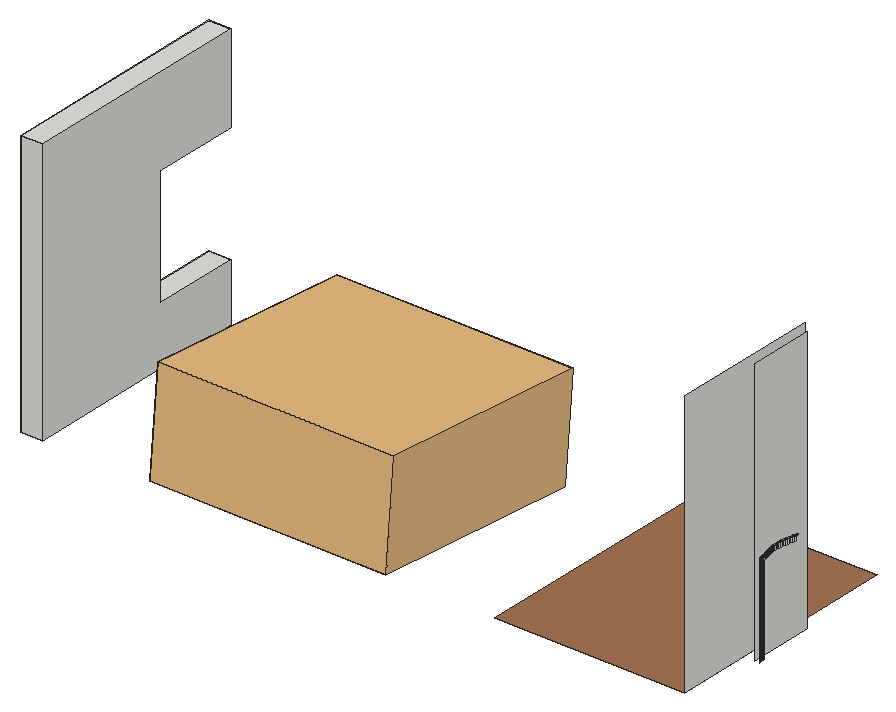
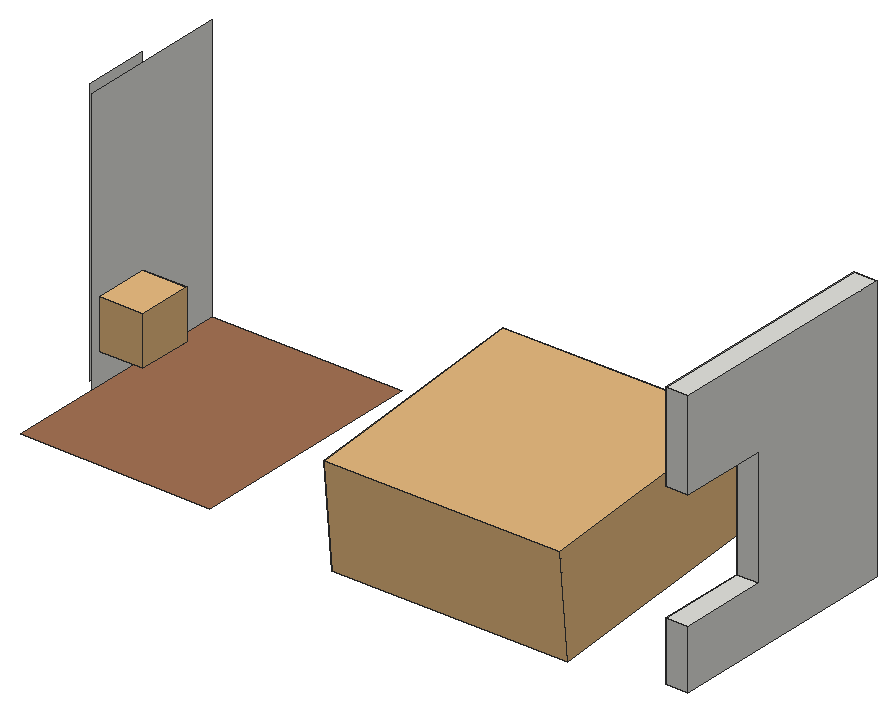
# SketchUp Ruby script. Lengths in inches.
U = 1.inch
M = Sketchup.active_model
def pt(a) = Geom::Point3d.new(a.map { |v| v * U })
def face(e, loops, mat)
  f = e.add_face(loops[0].map { |a| pt(a) })
  loops[1..].each { |l| e.add_face(l.map { |a| pt(a) }).erase! }
  f.material = f.back_material = mat if mat
  f
end
# faces: each face lists its corners as indices into pts; further lists are holes
def faces(e, pts, list, mat = nil) = list.each { |f| face(e, (f[0].is_a?(Array) ? f : [f]).map { |l| l.map { |i| pts[i] } }, mat) }
# xy, xz, yz: faces in a plane at the given z, y or x. An outline is a flat list of corners, or four numbers for a rectangle; further outlines are holes
def ring(l) = l.size == 4 ? [[l[0], l[1]], [l[2], l[1]], [l[2], l[3]], [l[0], l[3]]] : l.each_slice(2).to_a
def flat(e, list, mat, &to3) = list.each { |f| face(e, (f[0].is_a?(Array) ? f : [f]).map { |l| ring(l).map { |u, v| to3.(u, v) } }, mat) }
def xy(e, z, list, mat = nil) = flat(e, list, mat) { |x, y| [x, y, z] }
def xz(e, y, list, mat = nil) = flat(e, list, mat) { |x, z| [x, y, z] }
def yz(e, x, list, mat = nil) = flat(e, list, mat) { |y, z| [x, y, z] }
def lines(e, pts, list) = list.each { |a, b| e.add_line(pt(pts[a]), pt(pts[b])) }
# prism: a flat outline (further loops are holes) pulled along v
def prism(e, loops, v, mat = nil)
  f = face(e, loops, mat); d = Geom::Vector3d.new(v.map { |x| x * U })
  f.pushpull(f.normal.samedirection?(d) ? d.length : -d.length)
end
def box(e, o, s, mat = nil) = prism(e, [[o, [o[0] + s[0], o[1], o[2]], [o[0] + s[0], o[1] + s[1], o[2]], [o[0], o[1] + s[1], o[2]]]], [0, 0, s[2]], mat)
def at(x, y, z, deg = 0) = Geom::Transformation.translation(pt([x, y, z])) * Geom::Transformation.rotation(ORIGIN, Z_AXIS, deg.degrees)
def axes(o, x, y, z) = Geom::Transformation.new([*x, 0, *y, 0, *z, 0, *pt(o).to_a, 1])
def part(name) = M.definitions.add(name)
# library, detail: a bought-in or finely detailed component or shape, given as its bounding box
def library(name, o, s) = part(name).tap { |d| box(d.entities, o, s) }
def detail(e, o, s) = box(e.add_group.entities, o, s)
def put(e, d, t, mat = nil) = e.add_instance(d, t).tap { |i| i.material = mat if mat }
def group(e, t, mat = nil) = e.add_group.tap { |g| g.transformation = t; g.material = mat if mat }.entities
root = M.entities
M.materials.add("[Tile Ceramic Multi]").color = [165, 115, 84]
c1 = library("Kohler_lavatory_wellworth_sink",[0,0,-7.24],[22.26,18.23,19.81])
c2 = library("1.FBX",[-59.52,-60.59,0],[119.07,121.18,41.92])
xy(root,0,[[245.5,47.86,322.5,145.36]],"[Tile Ceramic Multi]")
yz(root,322.5,[[47.86,0,108.86,108]])
yz(root,327,[[78.05,0,104.36,108]])
yz(root,328.72,[[79.78,0,79.98,37.7],[79.98,0,80.18,37.7],[79.78,37.7,79.98,37.8],[79.98,37.7,80.18,37.8]])
p = [[329.13,77.74,0],[329.13,77.74,37.7],[329.06,77.85,37.7],[329.06,77.85,0],[329,77.96,37.7],[329,77.96,0],
  [328.95,78.08,37.7],[328.95,78.08,0],[328.96,78.05,0],[328.91,78.21,37.7],[328.91,78.21,0],[328.875,78.4,37.7],
  [328.875,78.4,0],[328.84,78.6,37.7],[328.84,78.6,0],[328.81,78.79,37.7],[328.81,78.79,0],[328.78,78.99,37.7],
  [328.78,78.99,0],[328.76,79.1875,37.7],[328.76,79.1875,0],[328.74,79.39,37.7],[328.74,79.39,0],[328.73,79.58,37.7],
  [328.73,79.58,0],[328.72,79.78,37.7],[328.72,79.78,0],[328.72,80.18,0],[328.72,80.18,37.7],[328.73,80.38,37.7],
  [328.73,80.38,0],[328.74,80.58,37.7],[328.74,80.58,35.76],[328.74,80.58,0],[328.52,81.27,37.7],[328.52,81.27,35.76],
  [328.31,81.96,37.7],[328.31,81.96,35.76],[328.12,82.66,37.7],[328.12,82.66,35.76],[327.94,83.37,37.7],[327.94,83.37,35.76],
  [327.78,84.07,37.7],[327.78,84.07,35.76],[327.625,84.78,37.7],[327.625,84.78,35.76],[327.49,85.5,37.7],[327.49,85.5,35.76],
  [327.36,86.21,37.7],[327.36,86.21,35.76],[327.25,86.93,37.7],[327.25,86.93,35.76],[327.15,87.65,37.7],[327.15,87.65,35.76],
  [327.07,88.37,37.7],[327.07,88.37,35.76],[327,89.09,37.7],[327,89.09,35.76],[327.07,89.82,37.7],[327.07,89.82,35.76],
  [327.15,90.54,37.7],[327.15,90.54,35.76],[327.25,91.26,37.7],[327.25,91.26,35.76],[327.36,91.97,37.7],[327.36,91.97,35.76],
  [327.49,92.6875,37.7],[327.49,92.6875,35.76],[327.625,93.4,37.7],[327.625,93.4,35.76],[327.78,94.11,37.7],[327.78,94.11,35.76],
  [327.94,94.82,37.7],[327.94,94.82,35.76],[328.12,95.52,37.7],[328.12,95.52,35.76],[328.31,96.22,37.7],[328.31,96.22,35.76],
  [328.52,96.92,37.7],[328.52,96.92,35.76],[329.21,77.65,37.8],[329.21,77.65,37.7],[329.13,77.75,37.8],[329.06,77.85,37.8],
  [329,77.97,37.8],[328.95,78.09,37.8],[328.92,78.21,37.8],[328.875,78.4,37.8],[328.84,78.6,37.8],[328.81,78.79,37.8],
  [328.78,78.99,37.8],[328.76,79.1875,37.8],[328.74,79.39,37.8],[328.73,79.58,37.8],[328.72,79.78,37.8],[328.72,80.18,37.8],
  [328.73,80.38,37.8],[328.74,80.58,37.8],[328.52,81.27,37.8],[328.32,81.97,37.8],[328.125,82.67,37.8],[327.95,83.37,37.8],
  [327.78,84.08,37.8],[327.63,84.79,37.8],[327.49,85.5,37.8],[327.37,86.21,37.8],[327.25,86.93,37.8],[327.16,87.65,37.8],
  [327.07,88.37,37.8],[327,89.09,37.8],[327.07,89.82,37.8],[327.16,90.54,37.8],[327.25,91.26,37.8],[327.37,91.97,37.8],
  [327.49,92.6875,37.8],[327.63,93.4,37.8],[327.78,94.11,37.8],[327.95,94.82,37.8],[328.125,95.52,37.8],[328.32,96.22,37.8],
  [328.52,96.92,37.8],[329.22,77.66,37.89],[329.14,77.75,37.89],[329.07,77.86,37.89],[329.01,77.97,37.89],[328.96,78.09,37.89],
  [328.93,78.21,37.89],[328.89,78.4,37.89],[328.85,78.6,37.89],[328.82,78.8,37.89],[328.79,78.99,37.89],[328.77,79.1875,37.89],
  [328.76,79.39,37.89],[328.74,79.58,37.89],[328.74,79.78,37.89],[328.72,79.98,37.8],[328.73,79.98,37.89],[328.74,80.18,37.89],
  [328.74,80.38,37.89],[328.76,80.58,37.89],[328.54,81.27,37.89],[328.33,81.97,37.89],[328.14,82.67,37.89],[327.96,83.37,37.89],
  [327.79,84.08,37.89],[327.64,84.79,37.89],[327.5,85.5,37.89],[327.375,86.21,37.89],[327.27,86.93,37.89],[327.17,87.65,37.89],
  [327.08,88.37,37.89],[327.01,89.09,37.89],[327.08,89.8125,37.89],[327.17,90.53,37.89],[327.27,91.25,37.89],[327.375,91.97,37.89],
  [327.5,92.6875,37.89],[327.64,93.4,37.89],[327.79,94.11,37.89],[327.96,94.8125,37.89],[328.14,95.52,37.89],[328.33,96.22,37.89],
  [328.54,96.91,37.89],[328.74,97.61,37.8],[328.76,97.61,37.89],[329.23,77.67,37.99],[329.15,77.76,37.99],[329.08,77.87,37.99],
  [329.03,77.98,37.99],[328.98,78.09,37.99],[328.95,78.22,37.99],[328.91,78.41,37.99],[328.87,78.6,37.99],[328.84,78.8,37.99],
  [328.8125,78.99,37.99],[328.79,79.19,37.99],[328.77,79.39,37.99],[328.76,79.59,37.99],[328.75,79.78,37.99],[328.75,79.98,37.99],
  [328.75,80.18,37.99],[328.76,80.375,37.99],[328.77,80.58,37.99],[328.55,81.28,37.99],[328.35,81.97,37.99],[328.15,82.67,37.99],
  [327.98,83.375,37.99],[327.81,84.08,37.99],[327.66,84.79,37.99],[327.52,85.5,37.99],[327.39,86.22,37.99],[327.28,86.93,37.99],
  [327.1875,87.65,37.99],[327.1,88.375,37.99],[327.03,89.09,37.99],[327.1,89.8125,37.99],[327.1875,90.53,37.99],[327.28,91.25,37.99],
  [327.39,91.97,37.99],[327.52,92.68,37.99],[327.66,93.39,37.99],[327.81,94.1,37.99],[327.98,94.81,37.99],[328.15,95.51,37.99],
  [328.35,96.21,37.99],[328.55,96.91,37.99],[328.77,97.61,37.99],[329.25,77.6875,38.08],[329.17,77.78,38.08],[329.11,77.88,38.08],
  [329.05,77.99,38.08],[329,78.1,38.08],[328.97,78.22,38.08],[328.93,78.41,38.08],[328.9,78.61,38.08],[328.86,78.8,38.08],
  [328.84,79,38.08],[328.82,79.19,38.08],[328.8,79.39,38.08],[328.79,79.59,38.08],[328.78,79.78,38.08],[328.78,79.98,38.08],
  [328.78,80.18,38.08],[328.79,80.375,38.08],[328.8,80.58,38.08],[328.58,81.29,38.08],[328.37,81.98,38.08],[328.18,82.68,38.08],
  [328,83.38,38.08],[327.84,84.09,38.08],[327.68,84.8,38.08],[327.54,85.51,38.08],[327.42,86.22,38.08],[327.31,86.9375,38.08],
  [327.21,87.66,38.08],[327.13,88.375,38.08],[327.06,89.09,38.08],[327.13,89.81,38.08],[327.21,90.53,38.08],[327.31,91.25,38.08],
  [327.42,91.96,38.08],[327.54,92.68,38.08],[327.68,93.39,38.08],[327.84,94.1,38.08],[328,94.8,38.08],[328.18,95.51,38.08],
  [328.37,96.21,38.08],[328.58,96.9,38.08],[328.8,97.6,38.08],[329.28,77.71,38.17],[329.2,77.8,38.17],[329.13,77.9,38.17],
  [329.08,78,38.17],[329.04,78.11,38.17],[329,78.23,38.17],[328.96,78.42,38.17],[328.93,78.61,38.17],[328.9,78.81,38.17],
  [328.87,79,38.17],[328.85,79.2,38.17],[328.83,79.39,38.17],[328.82,79.59,38.17],[328.8125,79.78,38.17],[328.8125,79.98,38.17],
  [328.8125,80.18,38.17],[328.82,80.375,38.17],[328.83,80.59,38.17],[328.61,81.3,38.17],[328.4,81.99,38.17],[328.21,82.6875,38.17],
  [328.03,83.39,38.17],[327.87,84.09,38.17],[327.72,84.8,38.17],[327.58,85.51,38.17],[327.45,86.23,38.17],[327.34,86.94,38.17],
  [327.24,87.66,38.17],[327.16,88.38,38.17],[327.09,89.09,38.17],[327.16,89.81,38.17],[327.24,90.53,38.17],[327.34,91.24,38.17],
  [327.45,91.96,38.17],[327.58,92.67,38.17],[327.72,93.38,38.17],[327.87,94.09,38.17],[328.03,94.8,38.17],[328.21,95.5,38.17],
  [328.4,96.2,38.17],[328.61,96.89,38.17],[328.83,97.6,38.17],[52.5,47.625,0],[52.5,143.86,0]]
faces(root,p,[[0,1,2,3],[3,2,4,5],[5,4,6,7,8],[7,6,9,10],[10,9,11,12],[12,11,13,14],[14,13,15,16],[16,15,17,18],
  [18,17,19,20],[20,19,21,22],[22,21,23,24],[24,23,25,26],[27,28,29,30],[30,29,31,32,33],[32,31,34,35],[35,34,36,37],
  [37,36,38,39],[39,38,40,41],[41,40,42,43],[43,42,44,45],[45,44,46,47],[47,46,48,49],[49,48,50,51],[51,50,52,53],
  [53,52,54,55],[55,54,56,57],[57,56,58,59],[59,58,60,61],[61,60,62,63],[63,62,64,65],[65,64,66,67],[67,66,68,69],
  [69,68,70,71],[71,70,72,73],[73,72,74,75],[75,74,76,77],[77,76,78,79],[80,81,1,82],[82,1,2,83],[83,2,4,84],
  [84,4,6,85],[85,6,9,86],[86,9,11,87],[87,11,13,88],[88,13,15,89],[89,15,17,90],[90,17,19,91],[91,19,21,92],
  [92,21,23,93],[93,23,25,94],[95,28,29,96],[96,29,31,97],[97,31,34,98],[98,34,36,99],[99,36,38,100],[100,38,40,101],
  [101,40,42,102],[102,42,44,103],[103,44,46,104],[104,46,48,105],[105,48,50,106],[106,50,52,107],[107,52,54,108],[108,54,56,109],
  [109,56,58,110],[110,58,60,111],[111,60,62,112],[112,62,64,113],[113,64,66,114],[114,66,68,115],[115,68,70,116],[116,70,72,117],
  [117,72,74,118],[118,74,76,119],[119,76,78,120],[121,80,82,122],[122,82,83,123],[123,83,84,124],[124,84,85,125],[125,85,86,126],
  [126,86,87,127],[127,87,88,128],[128,88,89,129],[129,89,90,130],[130,90,91,131],[131,91,92,132],[132,92,93,133],[133,93,94,134],
  [134,94,135,136],[136,135,95,137],[137,95,96,138],[138,96,97,139],[139,97,98,140],[140,98,99,141],[141,99,100,142],[142,100,101,143],
  [143,101,102,144],[144,102,103,145],[145,103,104,146],[146,104,105,147],[147,105,106,148],[148,106,107,149],[149,107,108,150],[150,108,109,151],
  [151,109,110,152],[152,110,111,153],[153,111,112,154],[154,112,113,155],[155,113,114,156],[156,114,115,157],[157,115,116,158],[158,116,117,159],
  [159,117,118,160],[160,118,119,161],[161,119,120,162],[162,120,163,164],[165,121,122,166],[166,122,123,167],[167,123,124,168],[168,124,125,169],
  [169,125,126,170],[170,126,127,171],[171,127,128,172],[172,128,129,173],[173,129,130,174],[174,130,131,175],[175,131,132,176],[176,132,133,177],
  [177,133,134,178],[178,134,136,179],[179,136,137,180],[180,137,138,181],[181,138,139,182],[182,139,140,183],[183,140,141,184],[184,141,142,185],
  [185,142,143,186],[186,143,144,187],[187,144,145,188],[188,145,146,189],[189,146,147,190],[190,147,148,191],[191,148,149,192],[192,149,150,193],
  [193,150,151,194],[194,151,152,195],[195,152,153,196],[196,153,154,197],[197,154,155,198],[198,155,156,199],[199,156,157,200],[200,157,158,201],
  [201,158,159,202],[202,159,160,203],[203,160,161,204],[204,161,162,205],[205,162,164,206],[207,165,166,208],[208,166,167,209],[209,167,168,210],
  [210,168,169,211],[211,169,170,212],[212,170,171,213],[213,171,172,214],[214,172,173,215],[215,173,174,216],[216,174,175,217],[217,175,176,218],
  [218,176,177,219],[219,177,178,220],[220,178,179,221],[221,179,180,222],[222,180,181,223],[223,181,182,224],[224,182,183,225],[225,183,184,226],
  [226,184,185,227],[227,185,186,228],[228,186,187,229],[229,187,188,230],[230,188,189,231],[231,189,190,232],[232,190,191,233],[233,191,192,234],
  [234,192,193,235],[235,193,194,236],[236,194,195,237],[237,195,196,238],[238,196,197,239],[239,197,198,240],[240,198,199,241],[241,199,200,242],
  [242,200,201,243],[243,201,202,244],[244,202,203,245],[245,203,204,246],[246,204,205,247],[247,205,206,248],[249,207,208,250],[250,208,209,251],
  [251,209,210,252],[252,210,211,253],[253,211,212,254],[254,212,213,255],[255,213,214,256],[256,214,215,257],[257,215,216,258],[258,216,217,259],
  [259,217,218,260],[260,218,219,261],[261,219,220,262],[262,220,221,263],[263,221,222,264],[264,222,223,265],[265,223,224,266],[266,224,225,267],
  [267,225,226,268],[268,226,227,269],[269,227,228,270],[270,228,229,271],[271,229,230,272],[272,230,231,273],[273,231,232,274],[274,232,233,275],
  [275,233,234,276],[276,234,235,277],[277,235,236,278],[278,236,237,279],[279,237,238,280],[280,238,239,281],[281,239,240,282],[282,240,241,283],
  [283,241,242,284],[284,242,243,285],[285,243,244,286],[286,244,245,287],[287,245,246,288],[288,246,247,289],[289,247,248,290]])
lines(root,p,[[291,292]])
put(root,c1,axes([304.52,105.68,20.17],[0.00001,-1,0],[1,0.00001,-0.00002],[0.00002,0,1]))
g1 = group(root,at(52.7,47.86,0))
prism(g1,[[[-0.1875,95.79,0],[-0.1875,0,0],[-0.1875,0,108],[-0.1875,95.73,108],[-0.1875,95.73,72],[-0.1875,59.79,72],[-0.1875,59.79,24],[-0.1875,95.79,24]]],[8.99,0,0])
put(root,c2,axes([152.04,94.64,-4.46],[-0.80514,-0.00151,0.00481],[0.00183,-0.75367,0.06983],[0.00578,0.09228,0.99572]))
